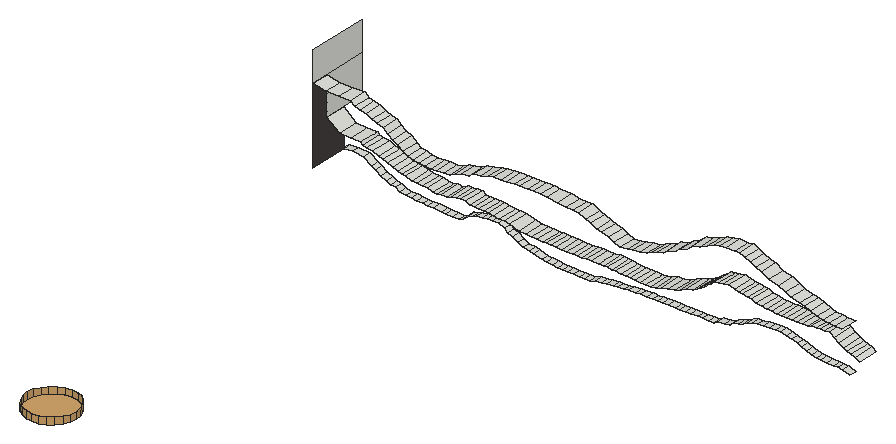
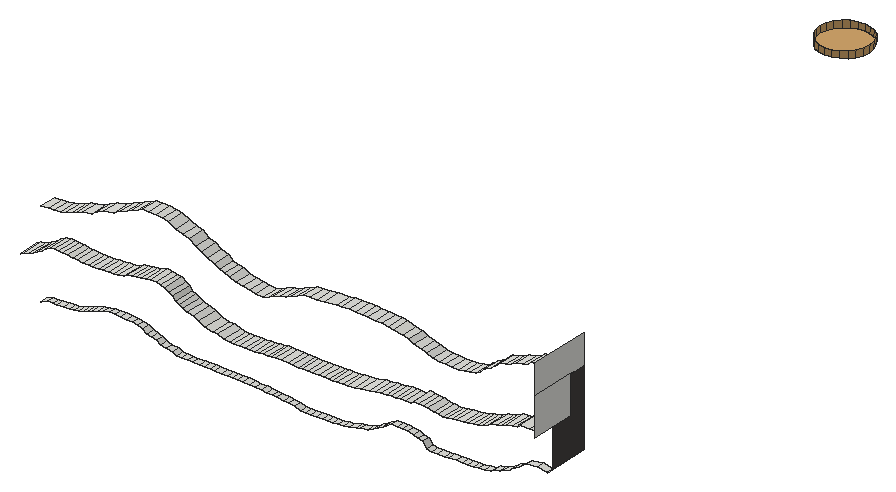
# SketchUp Ruby script. Lengths in inches.
U = 1.inch
M = Sketchup.active_model
def pt(a) = Geom::Point3d.new(a.map { |v| v * U })
def face(e, loops, mat)
  f = e.add_face(loops[0].map { |a| pt(a) })
  loops[1..].each { |l| e.add_face(l.map { |a| pt(a) }).erase! }
  f.material = f.back_material = mat if mat
  f
end
# faces: each face lists its corners as indices into pts; further lists are holes
def faces(e, pts, list, mat = nil) = list.each { |f| face(e, (f[0].is_a?(Array) ? f : [f]).map { |l| l.map { |i| pts[i] } }, mat) }
# xy, xz, yz: faces in a plane at the given z, y or x. An outline is a flat list of corners, or four numbers for a rectangle; further outlines are holes
def ring(l) = l.size == 4 ? [[l[0], l[1]], [l[2], l[1]], [l[2], l[3]], [l[0], l[3]]] : l.each_slice(2).to_a
def flat(e, list, mat, &to3) = list.each { |f| face(e, (f[0].is_a?(Array) ? f : [f]).map { |l| ring(l).map { |u, v| to3.(u, v) } }, mat) }
def xy(e, z, list, mat = nil) = flat(e, list, mat) { |x, y| [x, y, z] }
def xz(e, y, list, mat = nil) = flat(e, list, mat) { |x, z| [x, y, z] }
def yz(e, x, list, mat = nil) = flat(e, list, mat) { |y, z| [x, y, z] }
def lines(e, pts, list) = list.each { |a, b| e.add_line(pt(pts[a]), pt(pts[b])) }
# prism: a flat outline (further loops are holes) pulled along v
def prism(e, loops, v, mat = nil)
  f = face(e, loops, mat); d = Geom::Vector3d.new(v.map { |x| x * U })
  f.pushpull(f.normal.samedirection?(d) ? d.length : -d.length)
end
def box(e, o, s, mat = nil) = prism(e, [[o, [o[0] + s[0], o[1], o[2]], [o[0] + s[0], o[1] + s[1], o[2]], [o[0], o[1] + s[1], o[2]]]], [0, 0, s[2]], mat)
def at(x, y, z, deg = 0) = Geom::Transformation.translation(pt([x, y, z])) * Geom::Transformation.rotation(ORIGIN, Z_AXIS, deg.degrees)
def axes(o, x, y, z) = Geom::Transformation.new([*x, 0, *y, 0, *z, 0, *pt(o).to_a, 1])
def part(name) = M.definitions.add(name)
# library, detail: a bought-in or finely detailed component or shape, given as its bounding box
def library(name, o, s) = part(name).tap { |d| box(d.entities, o, s) }
def detail(e, o, s) = box(e.add_group.entities, o, s)
def put(e, d, t, mat = nil) = e.add_instance(d, t).tap { |i| i.material = mat if mat }
def group(e, t, mat = nil) = e.add_group.tap { |g| g.transformation = t; g.material = mat if mat }.entities
root = M.entities
M.materials.add("[Field Square Tile]").color = [211, 167, 108]
M.materials.add("[Granite Tile]1").color = [68, 65, 63]
xy(root,237.65,[[282.08,2401.37,282.77,2402.3],[282.77,2401.37,283.39,2402.3]])
xy(root,238.33,[[291.18,2401.37,291.73,2402.3],[291.73,2401.37,292.41,2402.3]])
xy(root,238.34,[[293.09,2401.37,294.02,2402.3],[294.02,2401.37,294.51,2402.3],[294.51,2401.37,295.27,2402.3],[295.27,2401.37,295.9,2402.3],[295.9,2401.37,296.65,2402.3],
  [296.65,2401.37,297.27,2402.3],[297.27,2401.37,298.04,2402.3],[298.04,2401.37,298.66,2402.3]])
xy(root,241.52,[[252.78,2396.68,252.84,2402.3]])
xy(root,241.68,[[283.28,2398.8,283.87,2401.37]])
xy(root,241.75,[[285.63,2398.8,286.5,2401.37],[286.5,2398.8,287.12,2401.37],[287.12,2398.8,287.63,2401.37]])
xy(root,250.6875,[[273.1,2327.89,272.31,2328,271.57,2328.3,270.93,2328.79,270.45,2329.43,270.14,2330.16,270.04,2330.96,270.14,2331.75,270.45,2332.49,270.93,2333.12,271.57,2333.61,272.31,2333.91,273.1,2334.02,273.89,2333.91,274.63,2333.61,275.26,2333.12,275.75,2332.49,276.06,2331.75,276.16,2330.96,276.06,2330.16,275.75,2329.43,275.26,2328.79,274.63,2328.3,273.89,2328]],"[Field Square Tile]")
xz(root,2396.68,[[252.78,241.52,252.84,251.5]])
yz(root,252.84,[[2398.8,246.2,2404.3,250.88],[2396.68,250.88,2404.3,254.5]])
yz(root,252.84,[[2396.68,241.52,2401.37,241.52,2401.37,246.2,2398.8,246.2,2398.8,250.88,2396.68,250.88]],"[Granite Tile]1")
p = [[283.39,2401.37,237.65],[283.39,2402.3,237.65],[284.06,2402.3,237.89],[284.06,2401.37,237.89],[278.72,2401.37,237.76],[278.72,2402.3,237.76],
  [279.43,2402.3,237.71],[279.43,2401.37,237.71],[280.04,2402.3,237.68],[280.04,2401.37,237.68],[280.64,2402.3,237.67],[280.64,2401.37,237.67],
  [281.39,2402.3,237.66],[281.39,2401.37,237.66],[282.08,2402.3,237.65],[282.08,2401.37,237.65],[277.37,2401.37,237.9],[277.37,2402.3,237.9],
  [278.03,2402.3,237.82],[278.03,2401.37,237.82],[276.43,2401.37,238.21],[276.43,2402.3,238.21],[284.82,2402.3,237.94],[284.82,2401.37,237.94],
  [285.4375,2402.3,237.98],[285.4375,2401.37,237.98],[286.29,2402.3,238.1],[286.29,2401.37,238.1],[286.84,2402.3,238.13],[286.84,2401.37,238.13],
  [287.6,2402.3,238.15],[287.6,2401.37,238.15],[275.96,2401.37,238.31],[275.96,2402.3,238.31],[288.23,2402.3,238.26],[288.23,2401.37,238.26],
  [275.05,2401.37,238.43],[275.05,2402.3,238.43],[288.98,2402.3,238.28],[288.98,2401.37,238.28],[289.61,2402.3,238.3],[289.61,2401.37,238.3],
  [290.46,2402.3,238.32],[290.46,2401.37,238.32],[291.18,2402.3,238.33],[291.18,2401.37,238.33],[292.41,2401.37,238.33],[292.41,2402.3,238.33],
  [293.09,2402.3,238.34],[293.09,2401.37,238.34],[298.66,2401.37,238.34],[298.66,2402.3,238.34],[299.17,2402.3,238.59],[299.17,2401.37,238.59],
  [274.4,2401.37,238.74],[274.4,2402.3,238.74],[314.69,2401.37,238.78],[314.69,2402.3,238.78],[315.47,2402.3,238.43],[315.47,2401.37,238.43],
  [299.99,2402.3,238.72],[299.99,2401.37,238.72],[273.82,2401.37,239.11],[273.82,2402.3,239.11],[300.68,2402.3,238.86],[300.68,2401.37,238.86],
  [264.03,2401.37,238.92],[264.03,2402.3,238.92],[265.07,2402.3,238.82],[265.07,2401.37,238.82],[265.58,2402.3,238.8],[265.58,2401.37,238.8],
  [266.45,2402.3,238.79],[266.45,2401.37,238.79],[267.19,2402.3,238.77],[267.19,2401.37,238.77],[267.72,2402.3,238.9375],[267.72,2401.37,238.9375],
  [311.97,2401.37,238.875],[311.97,2402.3,238.875],[312.72,2402.3,238.83],[312.72,2401.37,238.83],[313.48,2402.3,238.8],[313.48,2401.37,238.8],
  [314.02,2402.3,238.79],[314.02,2401.37,238.79],[261.94,2401.37,238.97],[261.94,2402.3,238.97],[262.64,2402.3,238.94],[262.64,2401.37,238.94],
  [263.34,2402.3,238.93],[263.34,2401.37,238.93],[268.28,2402.3,239.55],[268.28,2401.37,239.55],[301.19,2402.3,239.18],[301.19,2401.37,239.18],
  [310.82,2401.37,239.04],[310.82,2402.3,239.04],[311.4,2402.3,238.94],[311.4,2401.37,238.94],[260.57,2401.37,239.09],[260.57,2402.3,239.09],
  [261.26,2402.3,239.03],[261.26,2401.37,239.03],[310.16,2401.37,239.29],[310.16,2402.3,239.29],[259.79,2401.37,239.19],[259.79,2402.3,239.19],
  [273.24,2401.37,239.38],[273.24,2402.3,239.38],[259.28,2401.37,239.52],[259.28,2402.3,239.52],[301.78,2402.3,239.35],[301.78,2401.37,239.35],
  [309.58,2401.37,239.53],[309.58,2402.3,239.53],[272.78,2401.37,239.71],[272.78,2402.3,239.71],[302.34,2402.3,239.52],[302.34,2401.37,239.52],
  [258.72,2401.37,239.64],[258.72,2402.3,239.64],[302.89,2402.3,239.85],[302.89,2401.37,239.85],[309.05,2401.37,239.7],[309.05,2402.3,239.7],
  [258.27,2401.37,239.86],[258.27,2402.3,239.86],[268.86,2402.3,239.69],[268.86,2401.37,239.69],[269.41,2402.3,239.88],[269.41,2401.37,239.88],
  [272.08,2401.37,240.11],[272.08,2402.3,240.11],[308.36,2401.37,239.92],[308.36,2402.3,239.92],[303.53,2402.3,240.03],[303.53,2401.37,240.03],
  [257.48,2401.37,240.2],[257.48,2402.3,240.2],[270.14,2402.3,239.99],[270.14,2401.37,239.99],[307.73,2401.37,240.11],[307.73,2402.3,240.11],
  [270.73,2402.3,240.05],[270.73,2401.37,240.05],[271.39,2402.3,240.09],[271.39,2401.37,240.09],[304.1875,2402.3,240.12],[304.1875,2401.37,240.12],
  [304.86,2402.3,240.19],[304.86,2401.37,240.19],[306.95,2401.37,240.27],[306.95,2402.3,240.27],[256.88,2401.37,240.59],[256.88,2402.3,240.59],
  [305.625,2402.3,240.23],[305.625,2401.37,240.23],[306.33,2402.3,240.25],[306.33,2401.37,240.25],[256.34,2401.37,240.85],[256.34,2402.3,240.85],
  [255.32,2401.37,241.55],[255.32,2402.3,241.55],[289.26,2398.8,241.57],[289.26,2401.37,241.57],[289.8,2401.37,241.53],[289.8,2398.8,241.53],
  [290.42,2401.37,241.51],[290.42,2398.8,241.51],[290.97,2401.37,241.49],[290.97,2398.8,241.49],[291.67,2401.37,241.48],[291.67,2398.8,241.48],
  [292.33,2401.37,241.47],[292.33,2398.8,241.47],[292.9,2401.37,241.46],[292.9,2398.8,241.46],[293.61,2401.37,241.6],[293.61,2398.8,241.6],
  [252.84,2401.37,241.52],[252.84,2402.3,241.52],[254.05,2402.3,241.69],[254.05,2401.37,241.69],[288.65,2398.8,241.66],[288.65,2401.37,241.66],
  [294.34,2401.37,241.85],[294.34,2398.8,241.85],[279.62,2398.8,241.75],[279.62,2401.37,241.75],[280.07,2401.37,241.74],[280.07,2398.8,241.74],
  [280.62,2401.37,241.72],[280.62,2398.8,241.72],[281.25,2401.37,241.71],[281.25,2398.8,241.71],[281.88,2401.37,241.7],[281.88,2398.8,241.7],
  [282.61,2401.37,241.69],[282.61,2398.8,241.69],[283.28,2401.37,241.68],[283.28,2398.8,241.68],[283.87,2398.8,241.68],[283.87,2401.37,241.68],
  [284.36,2401.37,241.67],[284.36,2398.8,241.67],[285.0625,2401.37,241.74],[285.0625,2398.8,241.74],[285.63,2401.37,241.75],[285.63,2398.8,241.75],
  [287.63,2398.8,241.75],[287.63,2401.37,241.75],[288.12,2401.37,241.67],[288.12,2398.8,241.67],[277.43,2398.8,241.89],[277.43,2401.37,241.89],
  [278.25,2401.37,241.83],[278.25,2398.8,241.83],[278.85,2401.37,241.78],[278.85,2398.8,241.78],[295.01,2401.37,241.91],[295.01,2398.8,241.91],
  [276.66,2398.8,241.96],[276.66,2401.37,241.96],[295.91,2401.37,242.1],[295.91,2398.8,242.1],[275.49,2398.8,242.24],[275.49,2401.37,242.24],
  [296.68,2401.37,242.46],[296.68,2398.8,242.46],[274.82,2398.8,242.34],[274.82,2401.37,242.34],[318.29,2398.8,242.51],[318.29,2401.37,242.51],
  [318.8,2401.37,242.21],[318.8,2398.8,242.21],[274.16,2398.8,242.38],[274.16,2401.37,242.38],[273.5,2398.8,242.48],[273.5,2401.37,242.48],
  [265.32,2398.8,242.68],[265.32,2401.37,242.68],[265.99,2401.37,242.51],[265.99,2398.8,242.51],[266.51,2401.37,242.46],[266.51,2398.8,242.46],
  [267.05,2401.37,242.58],[267.05,2398.8,242.58],[272.86,2398.8,242.57],[272.86,2401.37,242.57],[297.38,2401.37,242.78],[297.38,2398.8,242.78],
  [317.7,2398.8,242.68],[317.7,2401.37,242.68],[267.68,2401.37,242.57],[267.68,2398.8,242.57],[268.31,2401.37,242.81],[268.31,2398.8,242.81],
  [270.08,2398.8,242.92],[270.08,2401.37,242.92],[270.51,2401.37,242.625],[270.51,2398.8,242.625],[271.12,2401.37,242.65],[271.12,2398.8,242.65],
  [271.67,2401.37,242.62],[271.67,2398.8,242.62],[272.3,2401.37,242.58],[272.3,2398.8,242.58],[263.97,2398.8,242.78],[263.97,2401.37,242.78],
  [264.78,2401.37,242.73],[264.78,2398.8,242.73],[317.2,2398.8,242.875],[317.2,2401.37,242.875],[262.67,2398.8,243.06],[262.67,2401.37,243.06],
  [263.39,2401.37,242.85],[263.39,2398.8,242.85],[268.88,2401.37,242.86],[268.88,2398.8,242.86],[298.15,2401.37,242.97],[298.15,2398.8,242.97],
  [269.44,2401.37,242.89],[269.44,2398.8,242.89],[316.81,2398.8,243.09],[316.81,2401.37,243.09],[298.68,2401.37,243.23],[298.68,2398.8,243.23],
  [261.6,2398.8,243.3],[261.6,2401.37,243.3],[262.1875,2401.37,243.14],[262.1875,2398.8,243.14],[316.2,2398.8,243.43],[316.2,2401.37,243.43],
  [299.08,2401.37,243.48],[299.08,2398.8,243.48],[260.96,2398.8,243.48],[260.96,2401.37,243.48],[315.66,2398.8,243.8],[315.66,2401.37,243.8],
  [260.44,2398.8,243.79],[260.44,2401.37,243.79],[299.6,2401.37,243.72],[299.6,2398.8,243.72],[299.9375,2401.37,244.12],[299.9375,2398.8,244.12],
  [259.78,2398.8,243.95],[259.78,2401.37,243.95],[315.06,2398.8,244.18],[315.06,2401.37,244.18],[259.26,2398.8,244.11],[259.26,2401.37,244.11],
  [307.88,2398.8,243.99],[307.88,2401.37,243.99],[308.6,2401.37,243.95],[308.6,2398.8,243.95],[309.1,2401.37,243.93],[309.1,2398.8,243.93],
  [309.79,2401.37,243.91],[309.79,2398.8,243.91],[310.36,2401.37,243.89],[310.36,2398.8,243.89],[311.06,2401.37,243.88],[311.06,2398.8,243.88],
  [311.71,2401.37,243.94],[311.71,2398.8,243.94],[312.35,2401.37,243.95],[312.35,2398.8,243.95],[312.91,2401.37,244.1],[312.91,2398.8,244.1],
  [306.7,2398.8,244.11],[306.7,2401.37,244.11],[307.26,2401.37,244.04],[307.26,2398.8,244.04],[258.59,2398.8,244.41],[258.59,2401.37,244.41],
  [300.41,2401.37,244.39],[300.41,2398.8,244.39],[305.95,2398.8,244.25],[305.95,2401.37,244.25],[313.54,2401.37,244.13],[313.54,2398.8,244.13],
  [314.02,2401.37,244.15],[314.02,2398.8,244.15],[314.54,2401.37,244.17],[314.54,2398.8,244.17],[305.49,2398.8,244.51],[305.49,2401.37,244.51],
  [257.83,2398.8,244.54],[257.83,2401.37,244.54],[300.89,2401.37,244.73],[300.89,2398.8,244.73],[257.27,2398.8,244.61],[257.27,2401.37,244.61],
  [304.34,2398.8,244.67],[304.34,2401.37,244.67],[304.95,2401.37,244.55],[304.95,2398.8,244.55],[257.05,2398.8,244.92],[257.05,2401.37,244.92],
  [301.375,2401.37,244.87],[301.375,2398.8,244.87],[303.29,2398.8,244.81],[303.29,2401.37,244.81],[303.86,2401.37,244.7],[303.86,2398.8,244.7],
  [302.64,2398.8,245.01],[302.64,2401.37,245.01],[254.41,2398.8,244.96],[254.41,2401.37,244.96],[255.8,2401.37,244.9375],[255.8,2398.8,244.9375],
  [301.96,2401.37,244.95],[301.96,2398.8,244.95],[252.84,2398.8,246.2],[252.84,2401.37,246.2],[290.09,2396.68,246.35],[290.09,2398.8,246.35],
  [290.86,2398.8,246.05],[290.86,2396.68,246.05],[291.76,2398.8,246.13],[291.76,2396.68,246.13],[292.47,2398.8,246.29],[292.47,2396.68,246.29],
  [293.27,2398.8,246.41],[293.27,2396.68,246.41],[289.48,2396.68,246.66],[289.48,2398.8,246.66],[294.18,2398.8,246.55],[294.18,2396.68,246.55],
  [265.9,2396.68,246.62],[265.9,2398.8,246.62],[266.64,2398.8,246.54],[266.64,2396.68,246.54],[267.42,2398.8,246.51],[267.42,2396.68,246.51],
  [268.2,2398.8,246.58],[268.2,2396.68,246.58],[317.39,2396.68,246.59],[317.39,2398.8,246.59],[318.28,2398.8,246.55],[318.28,2396.68,246.55],
  [265.24,2396.68,246.73],[265.24,2398.8,246.73],[269,2398.8,246.59],[269,2396.68,246.59],[269.8,2398.8,246.69],[269.8,2396.68,246.69],
  [294.91,2398.8,246.92],[294.91,2396.68,246.92],[316.68,2396.68,246.66],[316.68,2398.8,246.66],[264.52,2396.68,246.88],[264.52,2398.8,246.88],
  [270.51,2398.8,247.03],[270.51,2396.68,247.03],[288.625,2396.68,246.94],[288.625,2398.8,246.94],[315.89,2396.68,246.75],[315.89,2398.8,246.75],
  [315.2,2396.68,246.95],[315.2,2398.8,246.95],[263.97,2396.68,247.25],[263.97,2398.8,247.25],[287.94,2396.68,247.08],[287.94,2398.8,247.08],
  [295.52,2398.8,247.12],[295.52,2396.68,247.12],[271.2,2398.8,247.2],[271.2,2396.68,247.2],[314.39,2396.68,247.25],[314.39,2398.8,247.25],
  [287.26,2396.68,247.46],[287.26,2398.8,247.46],[296.2,2398.8,247.31],[296.2,2396.68,247.31],[272.17,2398.8,247.39],[272.17,2396.68,247.39],
  [313.71,2396.68,247.53],[313.71,2398.8,247.53],[263.33,2396.68,247.72],[263.33,2398.8,247.72],[296.77,2398.8,247.71],[296.77,2396.68,247.71],
  [272.8,2398.8,247.78],[272.8,2396.68,247.78],[286.63,2396.68,247.66],[286.63,2398.8,247.66],[313.13,2396.68,247.66],[313.13,2398.8,247.66],
  [262.68,2396.68,248.07],[262.68,2398.8,248.07],[285.79,2396.68,248.08],[285.79,2398.8,248.08],[297.7,2398.8,248.03],[297.7,2396.68,248.03],
  [312,2396.68,247.9],[312,2398.8,247.9],[273.58,2398.8,247.89],[273.58,2396.68,247.89],[274.58,2398.8,248.18],[274.58,2396.68,248.18],
  [311.4,2396.68,248.26],[311.4,2398.8,248.26],[298.41,2398.8,248.46],[298.41,2396.68,248.46],[262.05,2396.68,248.51],[262.05,2398.8,248.51],
  [284.17,2396.68,248.15],[284.17,2398.8,248.15],[284.99,2398.8,248.11],[284.99,2396.68,248.11],[275.22,2398.8,248.29],[275.22,2396.68,248.29],
  [283.14,2396.68,248.28],[283.14,2398.8,248.28],[276.11,2398.8,248.35],[276.11,2396.68,248.35],[281.74,2396.68,248.39],[281.74,2398.8,248.39],
  [310.49,2396.68,248.69],[310.49,2398.8,248.69],[276.84,2398.8,248.4],[276.84,2396.68,248.4],[277.83,2398.8,248.4375],[277.83,2396.68,248.4375],
  [278.49,2398.8,248.46],[278.49,2396.68,248.46],[281.01,2396.68,248.49],[281.01,2398.8,248.49],[261.56,2396.68,249.01],[261.56,2398.8,249.01],
  [279.38,2398.8,248.47],[279.38,2396.68,248.47],[280.12,2398.8,248.48],[280.12,2396.68,248.48],[299.19,2398.8,248.82],[299.19,2396.68,248.82],
  [309.27,2396.68,248.95],[309.27,2398.8,248.95],[299.91,2398.8,249.37],[299.91,2396.68,249.37],[308.38,2396.68,249.46],[308.38,2398.8,249.46],
  [260.79,2396.68,249.2],[260.79,2398.8,249.2],[260.12,2396.68,249.41],[260.12,2398.8,249.41],[259.45,2396.68,249.8],[259.45,2398.8,249.8],
  [300.7,2398.8,249.5625],[300.7,2396.68,249.5625],[307.62,2396.68,249.68],[307.62,2398.8,249.68],[301.6,2398.8,249.9],[301.6,2396.68,249.9],
  [306.96,2396.68,250.0625],[306.96,2398.8,250.0625],[258.65,2396.68,249.97],[258.65,2398.8,249.97],[302.52,2398.8,250.35],[302.52,2396.68,250.35],
  [258.04,2396.68,250.15],[258.04,2398.8,250.15],[257.51,2396.68,250.55],[257.51,2398.8,250.55],[306.27,2396.68,250.32],[306.27,2398.8,250.32],
  [303.18,2398.8,250.49],[303.18,2396.68,250.49],[305.65,2396.68,250.61],[305.65,2398.8,250.61],[252.84,2396.68,250.88],[252.84,2398.8,250.88],
  [254.43,2398.8,250.53],[254.43,2396.68,250.53],[256.05,2398.8,250.54],[256.05,2396.68,250.54],[303.99,2398.8,250.6],[303.99,2396.68,250.6],
  [305.01,2398.8,250.58],[305.01,2396.68,250.58],[273.1,2327.89,251.5],[272.31,2328,251.5],[272.31,2328,250.6875],[273.1,2327.89,250.6875],
  [273.89,2328,251.5],[273.89,2328,250.6875],[271.57,2328.3,251.5],[271.57,2328.3,250.6875],[274.63,2328.3,251.5],[274.63,2328.3,250.6875],
  [270.93,2328.79,251.5],[270.93,2328.79,250.6875],[275.26,2328.79,251.5],[275.26,2328.79,250.6875],[270.45,2329.43,251.5],[270.45,2329.43,250.6875],
  [275.75,2329.43,251.5],[275.75,2329.43,250.6875],[270.14,2330.16,251.5],[270.14,2330.16,250.6875],[276.06,2330.16,251.5],[276.06,2330.16,250.6875],
  [270.04,2330.96,251.5],[270.04,2330.96,250.6875],[276.16,2330.96,251.5],[276.16,2330.96,250.6875],[270.14,2331.75,251.5],[270.14,2331.75,250.6875],
  [276.06,2331.75,251.5],[276.06,2331.75,250.6875],[270.45,2332.49,251.5],[270.45,2332.49,250.6875],[275.75,2332.49,251.5],[275.75,2332.49,250.6875],
  [270.93,2333.12,251.5],[270.93,2333.12,250.6875],[275.26,2333.12,251.5],[275.26,2333.12,250.6875],[271.57,2333.61,251.5],[271.57,2333.61,250.6875],
  [274.63,2333.61,251.5],[274.63,2333.61,250.6875],[272.31,2333.91,251.5],[272.31,2333.91,250.6875],[273.89,2333.91,251.5],[273.89,2333.91,250.6875],
  [273.1,2334.02,251.5],[273.1,2334.02,250.6875]]
faces(root,p,[[0,1,2,3],[4,5,6,7],[7,6,8,9],[9,8,10,11],[11,10,12,13],[13,12,14,15],[16,17,18,19],[19,18,5,4],
  [20,21,17,16],[3,2,22,23],[23,22,24,25],[25,24,26,27],[27,26,28,29],[29,28,30,31],[32,33,21,20],[31,30,34,35],
  [36,37,33,32],[35,34,38,39],[39,38,40,41],[41,40,42,43],[43,42,44,45],[46,47,48,49],[50,51,52,53],[54,55,37,36],
  [56,57,58,59],[53,52,60,61],[62,63,55,54],[61,60,64,65],[66,67,68,69],[69,68,70,71],[71,70,72,73],[73,72,74,75],
  [75,74,76,77],[78,79,80,81],[81,80,82,83],[83,82,84,85],[85,84,57,56],[86,87,88,89],[89,88,90,91],[91,90,67,66],
  [77,76,92,93],[65,64,94,95],[96,97,98,99],[99,98,79,78],[100,101,102,103],[103,102,87,86],[104,105,97,96],[106,107,101,100],
  [108,109,63,62],[110,111,107,106],[95,94,112,113],[114,115,105,104],[116,117,109,108],[113,112,118,119],[120,121,111,110],[119,118,122,123],
  [124,125,115,114],[126,127,121,120],[93,92,128,129],[129,128,130,131],[132,133,117,116],[134,135,125,124],[123,122,136,137],[138,139,127,126],
  [131,130,140,141],[142,143,135,134],[141,140,144,145],[145,144,146,147],[137,136,148,149],[147,146,133,132],[149,148,150,151],[152,153,143,142],
  [154,155,139,138],[151,150,156,157],[157,156,158,159],[159,158,153,152],[160,161,155,154],[162,163,161,160],[164,165,166,167],[167,166,168,169],
  [169,168,170,171],[171,170,172,173],[173,172,174,175],[175,174,176,177],[177,176,178,179],[180,181,182,183],[184,185,165,164],[179,178,186,187],
  [183,182,163,162],[188,189,190,191],[191,190,192,193],[193,192,194,195],[195,194,196,197],[197,196,198,199],[199,198,200,201],[202,203,204,205],
  [205,204,206,207],[207,206,208,209],[210,211,212,213],[213,212,185,184],[214,215,216,217],[217,216,218,219],[219,218,189,188],[187,186,220,221],
  [222,223,215,214],[221,220,224,225],[226,227,223,222],[225,224,228,229],[230,231,227,226],[232,233,234,235],[236,237,231,230],[238,239,237,236],
  [240,241,242,243],[243,242,244,245],[245,244,246,247],[248,249,239,238],[229,228,250,251],[252,253,233,232],[247,246,254,255],[255,254,256,257],
  [258,259,260,261],[261,260,262,263],[263,262,264,265],[265,264,266,267],[267,266,249,248],[268,269,270,271],[271,270,241,240],[272,273,253,252],
  [274,275,276,277],[277,276,269,268],[257,256,278,279],[251,250,280,281],[279,278,282,283],[283,282,259,258],[284,285,273,272],[281,280,286,287],
  [288,289,290,291],[291,290,275,274],[292,293,285,284],[287,286,294,295],[296,297,289,288],[298,299,293,292],[300,301,297,296],[295,294,302,303],
  [303,302,304,305],[306,307,301,300],[308,309,299,298],[310,311,307,306],[312,313,314,315],[315,314,316,317],[317,316,318,319],[319,318,320,321],
  [321,320,322,323],[323,322,324,325],[325,324,326,327],[327,326,328,329],[330,331,332,333],[333,332,313,312],[334,335,311,310],[305,304,336,337],
  [338,339,331,330],[329,328,340,341],[341,340,342,343],[343,342,344,345],[345,344,309,308],[346,347,339,338],[348,349,335,334],[337,336,350,351],
  [352,353,349,348],[354,355,356,357],[357,356,347,346],[358,359,353,352],[351,350,360,361],[362,363,364,365],[365,364,355,354],[366,367,363,362],
  [368,369,370,371],[371,370,359,358],[361,360,372,373],[373,372,367,366],[374,375,369,368],[376,377,378,379],[379,378,380,381],[381,380,382,383],
  [383,382,384,385],[386,387,377,376],[385,384,388,389],[390,391,392,393],[393,392,394,395],[395,394,396,397],[398,399,400,401],[402,403,391,390],
  [397,396,404,405],[405,404,406,407],[389,388,408,409],[410,411,399,398],[412,413,403,402],[407,406,414,415],[416,417,387,386],[418,419,411,410],
  [420,421,419,418],[422,423,413,412],[424,425,417,416],[409,408,426,427],[415,414,428,429],[430,431,421,420],[432,433,425,424],[427,426,434,435],
  [429,428,436,437],[438,439,431,430],[440,441,423,422],[435,434,442,443],[437,436,444,445],[446,447,433,432],[448,449,439,438],[450,451,441,440],
  [452,453,447,446],[443,442,454,455],[456,457,449,448],[445,444,458,459],[459,458,460,461],[462,463,457,456],[455,454,464,465],[466,467,451,450],
  [468,469,470,471],[471,470,453,452],[461,460,472,473],[474,475,469,468],[473,472,476,477],[478,479,475,474],[480,481,463,462],[477,476,482,483],
  [483,482,484,485],[485,484,486,487],[488,489,479,478],[490,491,467,466],[487,486,492,493],[493,492,494,495],[495,494,489,488],[465,464,496,497],
  [498,499,481,480],[497,496,500,501],[502,503,499,498],[504,505,491,490],[506,507,505,504],[508,509,507,506],[501,500,510,511],[512,513,503,502],
  [511,510,514,515],[516,517,513,512],[518,519,509,508],[515,514,520,521],[522,523,519,518],[524,525,523,522],[526,527,517,516],[521,520,528,529],
  [530,531,527,526],[532,533,534,535],[535,534,536,537],[537,536,525,524],[529,528,538,539],[539,538,540,541],[541,540,531,530]])
faces(root,p,[[542,543,544,545],[546,542,545,547],[543,548,549,544],[550,546,547,551],[548,552,553,549],[554,550,551,555],[552,556,557,553],[558,554,555,559],
  [556,560,561,557],[562,558,559,563],[560,564,565,561],[566,562,563,567],[564,568,569,565],[570,566,567,571],[568,572,573,569],[574,570,571,575],
  [572,576,577,573],[578,574,575,579],[576,580,581,577],[582,578,579,583],[580,584,585,581],[586,582,583,587],[584,588,589,585],[588,586,587,589]],"[Field Square Tile]")
